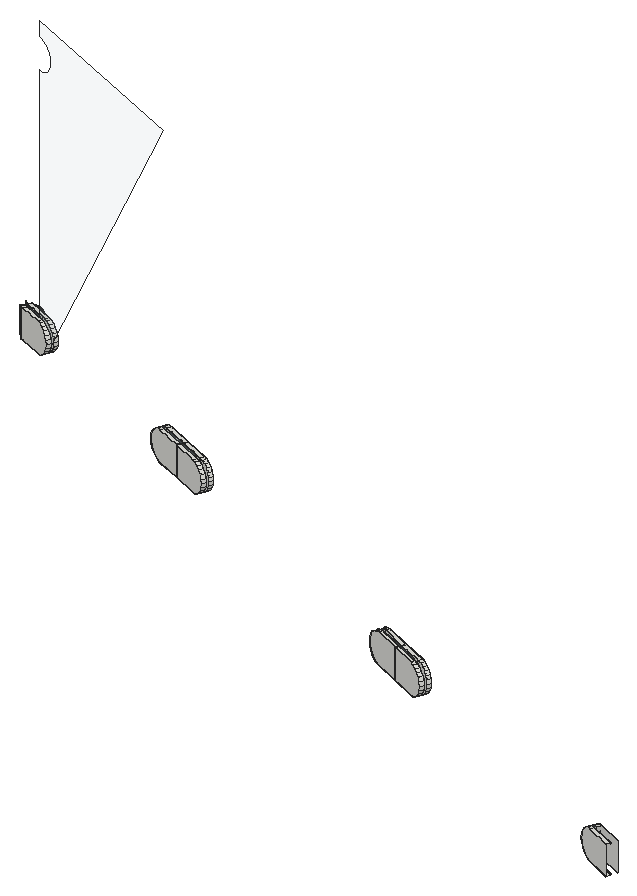
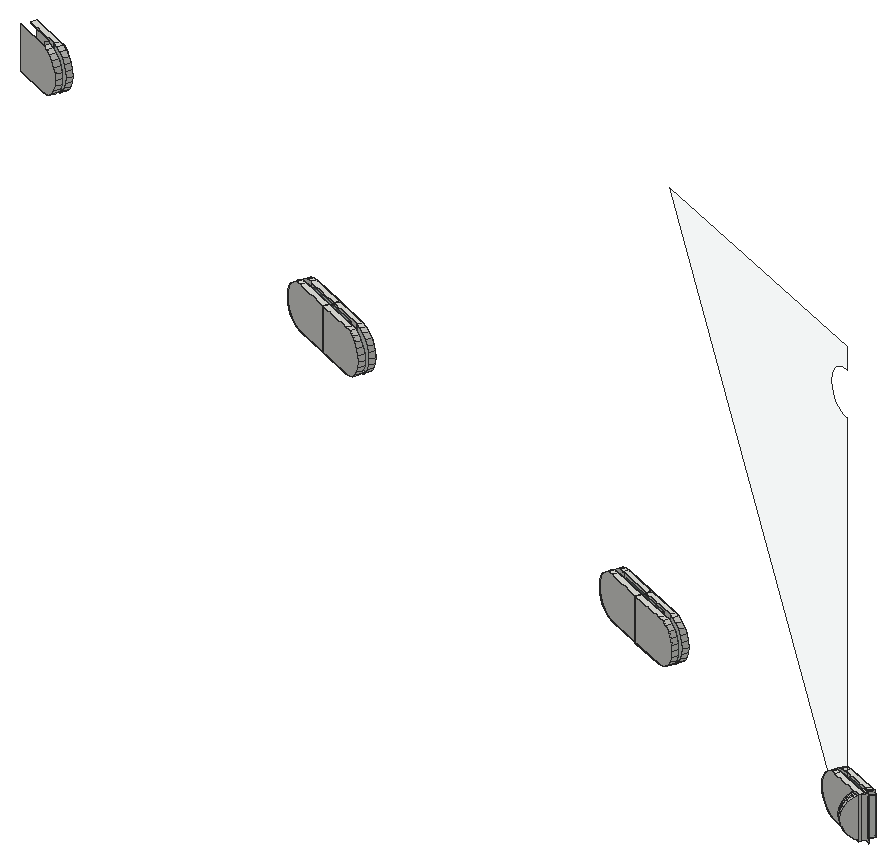
# SketchUp Ruby script. Lengths in inches.
U = 1.inch
M = Sketchup.active_model
def pt(a) = Geom::Point3d.new(a.map { |v| v * U })
def face(e, loops, mat)
  f = e.add_face(loops[0].map { |a| pt(a) })
  loops[1..].each { |l| e.add_face(l.map { |a| pt(a) }).erase! }
  f.material = f.back_material = mat if mat
  f
end
# faces: each face lists its corners as indices into pts; further lists are holes
def faces(e, pts, list, mat = nil) = list.each { |f| face(e, (f[0].is_a?(Array) ? f : [f]).map { |l| l.map { |i| pts[i] } }, mat) }
# xy, xz, yz: faces in a plane at the given z, y or x. An outline is a flat list of corners, or four numbers for a rectangle; further outlines are holes
def ring(l) = l.size == 4 ? [[l[0], l[1]], [l[2], l[1]], [l[2], l[3]], [l[0], l[3]]] : l.each_slice(2).to_a
def flat(e, list, mat, &to3) = list.each { |f| face(e, (f[0].is_a?(Array) ? f : [f]).map { |l| ring(l).map { |u, v| to3.(u, v) } }, mat) }
def xy(e, z, list, mat = nil) = flat(e, list, mat) { |x, y| [x, y, z] }
def xz(e, y, list, mat = nil) = flat(e, list, mat) { |x, z| [x, y, z] }
def yz(e, x, list, mat = nil) = flat(e, list, mat) { |y, z| [x, y, z] }
def lines(e, pts, list) = list.each { |a, b| e.add_line(pt(pts[a]), pt(pts[b])) }
# prism: a flat outline (further loops are holes) pulled along v
def prism(e, loops, v, mat = nil)
  f = face(e, loops, mat); d = Geom::Vector3d.new(v.map { |x| x * U })
  f.pushpull(f.normal.samedirection?(d) ? d.length : -d.length)
end
def box(e, o, s, mat = nil) = prism(e, [[o, [o[0] + s[0], o[1], o[2]], [o[0] + s[0], o[1] + s[1], o[2]], [o[0], o[1] + s[1], o[2]]]], [0, 0, s[2]], mat)
def at(x, y, z, deg = 0) = Geom::Transformation.translation(pt([x, y, z])) * Geom::Transformation.rotation(ORIGIN, Z_AXIS, deg.degrees)
def axes(o, x, y, z) = Geom::Transformation.new([*x, 0, *y, 0, *z, 0, *pt(o).to_a, 1])
def part(name) = M.definitions.add(name)
# library, detail: a bought-in or finely detailed component or shape, given as its bounding box
def library(name, o, s) = part(name).tap { |d| box(d.entities, o, s) }
def detail(e, o, s) = box(e.add_group.entities, o, s)
def put(e, d, t, mat = nil) = e.add_instance(d, t).tap { |i| i.material = mat if mat }
def group(e, t, mat = nil) = e.add_group.tap { |g| g.transformation = t; g.material = mat if mat }.entities
root = M.entities
M.materials.add("Glass_Safety_01").color = [204, 235, 244]
M.materials["Glass_Safety_01"].alpha = 0.1
xy(root,333,[[823.836,1099.203,822.031,1099.989,822.141,1100.242,823.946,1099.456],[802.031,1108.7,800.226,1109.486,800.336,1109.739,802.003,1109.013,802.141,1108.953],[802.22,1109.133,802.082,1109.193,800.415,1109.919,800.525,1110.172,802.33,1109.386],[800.226,1109.486,798.421,1110.272,798.531,1110.525,800.336,1109.739],[800.415,1109.919,798.61,1110.705,798.72,1110.958,800.525,1110.172],
  [777.687,1119.303,775.888,1120.086,775.994,1120.341,777.663,1119.614,777.797,1119.555],[777.876,1119.736,777.742,1119.794,776.071,1120.522,776.181,1120.775,777.986,1119.989],[775.888,1120.086,775.885,1120.087,775.882,1120.089,775.992,1120.341,775.994,1120.341],[775.882,1120.089,774.07,1120.841,774.176,1121.095,775.992,1120.341],[776.069,1120.523,774.251,1121.277,774.357,1121.532,776.175,1120.777],
  [760.716,1126.381,759.144,1127.034,759.32,1127.233,759.338,1127.252,760.627,1126.717,760.822,1126.636],[760.897,1126.818,760.702,1126.899,759.079,1127.572,759.184,1127.827,761.003,1127.072],[759.144,1127.034,758.951,1127.114,759.145,1127.332,759.265,1127.282,759.32,1127.233],[758.951,1127.114,758.898,1127.136,758.926,1127.204,759.068,1127.364,759.145,1127.332],[758.926,1127.204,759.003,1127.39,759.068,1127.364],
  [759.32,1127.233,759.265,1127.282,759.338,1127.252],[759.338,1127.252,759.265,1127.282,759.173,1127.364,759.195,1127.388,759.342,1127.257],[759.265,1127.282,759.145,1127.332,759.173,1127.364]])
xy(root,333.078,[[801.78,1109.11,800.336,1109.739,800.415,1109.919,801.859,1109.291],[800.336,1109.739,798.892,1110.368,798.971,1110.548,800.415,1109.919],[777.436,1119.713,775.994,1120.341,776.032,1120.432,776.071,1120.522,777.515,1119.893],[775.992,1120.341,774.539,1120.944,774.615,1121.126,776.069,1120.523,776.032,1120.432],[775.992,1120.341,776.032,1120.432,775.994,1120.341],
  [760.458,1126.787,759.068,1127.364,759.115,1127.416,759.041,1127.481,759.079,1127.572,760.533,1126.969],[758.875,1127.146,758.728,1127.277,758.968,1127.547,759.041,1127.481,759.003,1127.39,759.068,1127.364],[759.068,1127.364,759.003,1127.39,759.041,1127.481,759.115,1127.416]],"Glass_Safety_01")
xy(root,335.047,[[801.78,1109.11,801.859,1109.291,800.415,1109.919,800.336,1109.739],[800.336,1109.739,800.415,1109.919,798.971,1110.548,798.892,1110.368],[777.436,1119.713,777.515,1119.893,776.071,1120.522,776.032,1120.432,775.994,1120.341],[775.992,1120.341,776.032,1120.432,776.069,1120.523,774.615,1121.126,774.539,1120.944],[775.992,1120.341,775.994,1120.341,776.032,1120.432],
  [760.458,1126.787,760.533,1126.969,759.079,1127.572,759.041,1127.481,759.115,1127.416,759.068,1127.364],[758.875,1127.146,759.068,1127.364,759.003,1127.39,759.041,1127.481,758.968,1127.547,758.728,1127.277],[759.068,1127.364,759.115,1127.416,759.041,1127.481,759.003,1127.39]],"Glass_Safety_01")
xy(root,335.125,[[823.836,1099.203,823.946,1099.456,822.141,1100.242,822.031,1099.989],[802.031,1108.7,802.141,1108.953,802.003,1109.013,800.336,1109.739,800.226,1109.486],[802.22,1109.133,802.33,1109.386,800.525,1110.172,800.415,1109.919,802.082,1109.193],[800.226,1109.486,800.336,1109.739,798.531,1110.525,798.421,1110.272],[800.415,1109.919,800.525,1110.172,798.72,1110.958,798.61,1110.705],
  [777.687,1119.303,777.797,1119.555,777.663,1119.614,775.994,1120.341,775.888,1120.086],[777.876,1119.736,777.986,1119.989,776.181,1120.775,776.071,1120.522,777.742,1119.794],[775.888,1120.086,775.994,1120.341,775.992,1120.341,775.882,1120.089,775.885,1120.087],[775.882,1120.089,775.992,1120.341,774.176,1121.095,774.07,1120.841],[776.069,1120.523,776.175,1120.777,774.357,1121.532,774.251,1121.277],
  [760.716,1126.381,760.822,1126.636,760.627,1126.717,759.338,1127.252,759.32,1127.233,759.144,1127.034],[760.897,1126.818,761.003,1127.072,759.184,1127.827,759.079,1127.572,760.702,1126.899],[759.144,1127.034,759.32,1127.233,759.265,1127.282,759.145,1127.332,758.951,1127.114],[758.951,1127.114,759.145,1127.332,759.068,1127.364,758.926,1127.204,758.898,1127.136],[758.926,1127.204,759.068,1127.364,759.003,1127.39],
  [759.32,1127.233,759.338,1127.252,759.265,1127.282],[759.338,1127.252,759.342,1127.257,759.195,1127.388,759.173,1127.364,759.265,1127.282],[759.265,1127.282,759.173,1127.364,759.145,1127.332]])
xz(root,1120.341,[[775.992,333,775.994,333.078],[775.992,333.078,775.994,335.047],[775.992,333.078,775.994,335.125],[775.992,335.047,775.994,335.125]])
p = [[823.836,1099.203,335.125],[822.031,1099.989,335.125],[821.779,1100.099,335.089],[821.544,1100.202,334.983],[821.342,1100.29,334.814],[821.1875,1100.357,334.594],
  [821.09,1100.399,334.338],[821.057,1100.414,334.0625],[821.09,1100.399,333.787],[821.1875,1100.357,333.531],[821.342,1100.29,333.311],[821.544,1100.202,333.142],
  [821.779,1100.099,333.036],[822.031,1099.989,333],[823.836,1099.203,333],[823.946,1099.456,333],[822.141,1100.242,333],[822.141,1100.242,335.125],
  [823.946,1099.456,335.125],[823.946,1099.456,335.047],[822.502,1100.085,335.047],[822.502,1100.085,333.078],[823.946,1099.456,333.078],[822.33,1100.675,335.125],
  [824.135,1099.889,335.125],[824.135,1099.889,333],[822.33,1100.675,333],[822.078,1100.785,333.036],[821.843,1100.887,333.142],[821.641,1100.975,333.311],
  [821.486,1101.043,333.531],[821.389,1101.085,333.787],[821.355,1101.1,334.0625],[821.389,1101.085,334.338],[821.486,1101.043,334.594],[821.641,1100.975,334.814],
  [821.843,1100.887,334.983],[822.078,1100.785,335.089],[821.889,1100.352,333.036],[821.654,1100.454,333.142],[821.889,1100.352,335.089],[821.654,1100.454,334.983],
  [821.452,1100.542,334.814],[821.297,1100.61,334.594],[821.2,1100.652,334.338],[821.167,1100.667,334.0625],[821.2,1100.652,333.787],[821.297,1100.61,333.531],
  [821.452,1100.542,333.311],[822.22,1100.423,335.125],[822.22,1100.423,333],[821.968,1100.532,333.036],[821.733,1100.635,333.142],[821.531,1100.723,333.311],
  [821.376,1100.79,333.531],[821.279,1100.833,333.787],[821.245,1100.847,334.0625],[821.279,1100.833,334.338],[821.376,1100.79,334.594],[821.531,1100.723,334.814],
  [821.733,1100.635,334.983],[821.968,1100.532,335.089],[802.031,1108.7,335.125],[800.226,1109.486,335.125],[800.226,1109.486,333],[802.031,1108.7,333],
  [802.283,1108.59,333.036],[802.518,1108.488,333.142],[802.72,1108.4,333.311],[802.875,1108.333,333.531],[802.972,1108.29,333.787],[803.006,1108.276,334.0625],
  [802.972,1108.29,334.338],[802.875,1108.333,334.594],[802.72,1108.4,334.814],[802.518,1108.488,334.983],[802.283,1108.59,335.089],[802.141,1108.953,333],
  [802.003,1109.013,333],[802.003,1109.013,335.125],[802.141,1108.953,335.125],[802.393,1108.843,335.089],[802.628,1108.741,334.983],[802.83,1108.653,334.814],
  [802.985,1108.585,334.594],[803.082,1108.543,334.338],[803.116,1108.528,334.0625],[803.082,1108.543,333.787],[802.985,1108.585,333.531],[802.83,1108.653,333.311],
  [802.628,1108.741,333.142],[802.393,1108.843,333.036],[802.22,1109.133,335.125],[802.082,1109.193,335.125],[802.082,1109.193,333],[802.22,1109.133,333],
  [802.472,1109.023,333.036],[802.707,1108.921,333.142],[802.909,1108.833,333.311],[803.064,1108.766,333.531],[803.161,1108.723,333.787],[803.194,1108.709,334.0625],
  [803.161,1108.723,334.338],[803.064,1108.766,334.594],[802.909,1108.833,334.814],[802.707,1108.921,334.983],[802.472,1109.023,335.089],[802.582,1109.276,333.036],
  [802.817,1109.174,333.142],[800.336,1109.739,335.125],[800.336,1109.739,333],[800.336,1109.739,333.078],[801.78,1109.11,333.078],[801.78,1109.11,335.047],
  [800.336,1109.739,335.047],[800.525,1110.172,335.125],[802.33,1109.386,335.125],[802.582,1109.276,335.089],[802.817,1109.174,334.983],[803.019,1109.086,334.814],
  [803.174,1109.018,334.594],[803.271,1108.976,334.338],[803.304,1108.962,334.0625],[803.271,1108.976,333.787],[803.174,1109.018,333.531],[803.019,1109.086,333.311],
  [802.33,1109.386,333],[800.525,1110.172,333],[800.415,1109.919,333],[800.415,1109.919,335.125],[800.415,1109.919,335.047],[801.859,1109.291,335.047],
  [801.859,1109.291,333.078],[800.415,1109.919,333.078],[798.421,1110.272,335.125],[798.169,1110.382,335.089],[797.934,1110.484,334.983],[797.732,1110.572,334.814],
  [797.577,1110.64,334.594],[797.48,1110.682,334.338],[797.447,1110.697,334.0625],[797.48,1110.682,333.787],[797.577,1110.64,333.531],[797.732,1110.572,333.311],
  [797.934,1110.484,333.142],[798.169,1110.382,333.036],[798.421,1110.272,333],[798.531,1110.525,333],[798.531,1110.525,335.125],[798.892,1110.368,335.047],
  [798.892,1110.368,333.078],[798.61,1110.705,335.125],[798.61,1110.705,333],[798.971,1110.548,333.078],[798.971,1110.548,335.047],[798.72,1110.958,335.125],
  [798.72,1110.958,333],[798.468,1111.068,333.036],[798.233,1111.17,333.142],[798.031,1111.258,333.311],[797.876,1111.326,333.531],[797.779,1111.368,333.787],
  [797.746,1111.382,334.0625],[797.779,1111.368,334.338],[797.876,1111.326,334.594],[798.031,1111.258,334.814],[798.233,1111.17,334.983],[798.468,1111.068,335.089],
  [798.279,1110.635,333.036],[798.044,1110.737,333.142],[798.279,1110.635,335.089],[798.044,1110.737,334.983],[797.842,1110.825,334.814],[797.6875,1110.892,334.594],
  [797.59,1110.935,334.338],[797.557,1110.949,334.0625],[797.59,1110.935,333.787],[797.6875,1110.892,333.531],[797.842,1110.825,333.311],[798.358,1110.815,333.036],
  [798.123,1110.918,333.142],[797.921,1111.005,333.311],[797.766,1111.073,333.531],[797.669,1111.115,333.787],[797.636,1111.13,334.0625],[797.669,1111.115,334.338],
  [797.766,1111.073,334.594],[797.921,1111.005,334.814],[798.123,1110.918,334.983],[798.358,1110.815,335.089],[777.687,1119.303,335.125],[775.888,1120.086,335.125],
  [775.888,1120.086,333],[777.687,1119.303,333],[777.939,1119.193,333.036],[778.174,1119.09,333.142],[778.376,1119.003,333.311],[778.531,1118.935,333.531],
  [778.628,1118.893,333.787],[778.662,1118.878,334.0625],[778.628,1118.893,334.338],[778.531,1118.935,334.594],[778.376,1119.003,334.814],[778.174,1119.09,334.983],
  [777.939,1119.193,335.089],[777.797,1119.555,333],[777.663,1119.614,333],[777.663,1119.614,335.125],[777.797,1119.555,335.125],[778.049,1119.446,335.089],
  [778.284,1119.343,334.983],[778.486,1119.255,334.814],[778.641,1119.188,334.594],[778.738,1119.145,334.338],[778.772,1119.131,334.0625],[778.738,1119.145,333.787],
  [778.641,1119.188,333.531],[778.486,1119.255,333.311],[778.284,1119.343,333.142],[778.049,1119.446,333.036],[777.876,1119.736,335.125],[777.742,1119.794,335.125],
  [777.742,1119.794,333],[777.876,1119.736,333],[778.128,1119.626,333.036],[778.363,1119.524,333.142],[778.565,1119.436,333.311],[778.72,1119.368,333.531],
  [778.817,1119.326,333.787],[778.85,1119.311,334.0625],[778.817,1119.326,334.338],[778.72,1119.368,334.594],[778.565,1119.436,334.814],[778.363,1119.524,334.983],
  [778.128,1119.626,335.089],[778.238,1119.879,333.036],[778.473,1119.776,333.142],[775.994,1120.341,335.125],[775.994,1120.341,333],[775.994,1120.341,333.078],
  [777.436,1119.713,333.078],[777.436,1119.713,335.047],[775.994,1120.341,335.047],[776.181,1120.775,335.125],[777.986,1119.989,335.125],[778.238,1119.879,335.089],
  [778.473,1119.776,334.983],[778.675,1119.688,334.814],[778.83,1119.621,334.594],[778.927,1119.579,334.338],[778.96,1119.564,334.0625],[778.927,1119.579,333.787],
  [778.83,1119.621,333.531],[778.675,1119.688,333.311],[777.986,1119.989,333],[776.181,1120.775,333],[776.071,1120.522,333],[776.071,1120.522,335.125],
  [776.071,1120.522,335.047],[777.515,1119.893,335.047],[777.515,1119.893,333.078],[776.071,1120.522,333.078],[775.885,1120.087,335.125],[775.882,1120.089,335.125],
  [774.07,1120.841,335.125],[773.816,1120.946,335.089],[773.579,1121.044,334.983],[773.376,1121.129,334.814],[773.22,1121.193,334.594],[773.122,1121.234,334.338],
  [773.088,1121.248,334.0625],[773.122,1121.234,333.787],[773.22,1121.193,333.531],[773.376,1121.129,333.311],[773.579,1121.044,333.142],[773.816,1120.946,333.036],
  [774.07,1120.841,333],[775.882,1120.089,333],[775.885,1120.087,333],[775.992,1120.341,333.078],[775.992,1120.341,333],[775.992,1120.341,335.125],
  [775.992,1120.341,335.047],[774.176,1121.095,333],[774.176,1121.095,335.125],[774.539,1120.944,335.047],[774.539,1120.944,333.078],[776.069,1120.523,335.125],
  [774.251,1121.277,335.125],[774.251,1121.277,333],[776.069,1120.523,333],[776.069,1120.523,333.078],[774.615,1121.126,333.078],[774.615,1121.126,335.047],
  [776.069,1120.523,335.047],[776.175,1120.777,333],[776.175,1120.777,335.125],[774.357,1121.532,335.125],[774.357,1121.532,333],[774.103,1121.637,333.036],
  [773.866,1121.735,333.142],[773.662,1121.82,333.311],[773.506,1121.884,333.531],[773.408,1121.925,333.787],[773.375,1121.939,334.0625],[773.408,1121.925,334.338],
  [773.506,1121.884,334.594],[773.662,1121.82,334.814],[773.866,1121.735,334.983],[774.103,1121.637,335.089],[773.922,1121.201,333.036],[773.685,1121.299,333.142],
  [773.922,1121.201,335.089],[773.685,1121.299,334.983],[773.481,1121.383,334.814],[773.325,1121.448,334.594],[773.227,1121.489,334.338],[773.194,1121.503,334.0625],
  [773.227,1121.489,333.787],[773.325,1121.448,333.531],[773.481,1121.383,333.311],[773.997,1121.382,333.036],[773.76,1121.481,333.142],[773.557,1121.565,333.311],
  [773.401,1121.63,333.531],[773.303,1121.67,333.787],[773.269,1121.684,334.0625],[773.303,1121.67,334.338],[773.401,1121.63,334.594],[773.557,1121.565,334.814],
  [773.76,1121.481,334.983],[773.997,1121.382,335.089],[758.951,1127.114,335.125],[758.898,1127.136,335.125],[758.898,1127.136,333],[758.951,1127.114,333],
  [759.144,1127.034,333],[760.716,1126.381,333],[760.97,1126.276,333.036],[761.207,1126.178,333.142],[761.41,1126.093,333.311],[761.566,1126.029,333.531],
  [761.664,1125.988,333.787],[761.698,1125.974,334.0625],[761.664,1125.988,334.338],[761.566,1126.029,334.594],[761.41,1126.093,334.814],[761.207,1126.178,334.983],
  [760.97,1126.276,335.089],[760.716,1126.381,335.125],[759.144,1127.034,335.125],[761.773,1126.241,333.809],[761.433,1126.383,333.242],[761.3125,1126.432,333.142],
  [761.076,1126.531,333.036],[760.822,1126.636,333],[760.627,1126.717,333],[760.627,1126.717,335.125],[760.822,1126.636,335.125],[761.076,1126.531,335.089],
  [761.3125,1126.432,334.983],[761.516,1126.348,334.814],[761.672,1126.283,334.594],[761.77,1126.243,334.338],[761.803,1126.229,334.0625],[760.897,1126.818,335.125],
  [760.702,1126.899,335.125],[760.702,1126.899,333],[760.897,1126.818,333],[761.151,1126.712,333.036],[761.388,1126.614,333.142],[761.591,1126.53,333.311],
  [761.747,1126.465,333.531],[761.845,1126.424,333.787],[761.879,1126.41,334.0625],[761.845,1126.424,334.338],[761.747,1126.465,334.594],[761.591,1126.53,334.814],
  [761.388,1126.614,334.983],[761.151,1126.712,335.089],[761.257,1126.967,333.036],[761.494,1126.869,333.142],[759.338,1127.252,335.125],[759.338,1127.252,333],
  [759.265,1127.282,333],[759.145,1127.332,333],[759.068,1127.364,333],[759.003,1127.39,333],[759.003,1127.39,333.078],[759.068,1127.364,333.078],
  [760.458,1126.787,333.078],[760.458,1126.787,335.047],[759.068,1127.364,335.047],[759.003,1127.39,335.047],[759.003,1127.39,335.125],[759.068,1127.364,335.125],
  [759.145,1127.332,335.125],[759.265,1127.282,335.125],[759.184,1127.827,335.125],[761.003,1127.072,335.125],[761.257,1126.967,335.089],[761.494,1126.869,334.983],
  [761.697,1126.784,334.814],[761.853,1126.72,334.594],[761.951,1126.679,334.338],[761.984,1126.665,334.0625],[761.951,1126.679,333.787],[761.853,1126.72,333.531],
  [761.697,1126.784,333.311],[761.003,1127.072,333],[759.184,1127.827,333],[759.079,1127.572,333],[759.079,1127.572,335.125],[759.079,1127.572,335.047],
  [760.533,1126.969,335.047],[760.533,1126.969,333.078],[759.079,1127.572,333.078],[758.926,1127.204,333],[758.926,1127.204,335.125],[759.115,1127.416,333],
  [759.115,1127.416,333.078],[759.115,1127.416,335.047],[759.115,1127.416,335.125],[759.173,1127.364,335.125],[759.32,1127.233,335.125],[759.32,1127.233,333],
  [759.173,1127.364,333],[759.342,1127.257,335.125],[759.525,1127.463,335.089],[759.696,1127.654,334.983],[759.842,1127.819,334.814],[759.954,1127.945,334.594],
  [760.025,1128.024,334.338],[760.049,1128.051,334.0625],[760.025,1128.024,333.787],[759.954,1127.945,333.531],[759.842,1127.819,333.311],[759.696,1127.654,333.142],
  [759.525,1127.463,333.036],[759.342,1127.257,333],[759.378,1127.594,333.036],[759.195,1127.388,333],[758.989,1127.571,333],[759.172,1127.777,333.036],
  [759.319,1127.646,333.036],[759.136,1127.44,333],[758.968,1127.547,333.078],[758.968,1127.547,333],[758.762,1127.73,333],[758.762,1127.73,335.125],
  [758.968,1127.547,335.125],[758.968,1127.547,335.047],[758.989,1127.571,335.125],[759.172,1127.777,335.089],[759.343,1127.968,334.983],[759.489,1128.133,334.814],
  [759.602,1128.259,334.594],[759.672,1128.338,334.338],[759.696,1128.365,334.0625],[759.672,1128.338,333.787],[759.602,1128.259,333.531],[759.489,1128.133,333.311],
  [759.343,1127.968,333.142],[759.549,1127.785,333.142],[759.49,1127.837,333.142],[822.581,1100.265,335.047],[822.581,1100.265,333.078],[776.032,1120.432,335.047],
  [776.032,1120.432,333.078],[761.516,1126.348,333.311],[758.728,1127.277,333.078],[758.728,1127.277,335.047],[758.875,1127.146,335.047],[758.875,1127.146,333.078],
  [759.041,1127.481,335.047],[759.041,1127.481,333.078],[759.695,1127.949,333.311],[759.636,1128.002,333.311],[761.77,1126.243,333.787],[761.672,1126.283,333.531],
  [759.807,1128.076,333.531],[759.749,1128.128,333.531],[759.878,1128.155,333.787],[759.819,1128.207,333.787],[760.627,1126.717,351.283],[774.176,1121.095,354.511],
  [760.627,1126.717,354.511],[760.627,1126.717,353.409],[760.822,1126.636,353.409],[761.076,1126.531,353.373],[761.3125,1126.432,353.267],[761.516,1126.348,353.098],
  [761.672,1126.283,352.877],[761.77,1126.243,352.621],[761.803,1126.229,352.346],[761.77,1126.243,352.071],[761.672,1126.283,351.814],[761.516,1126.348,351.594],
  [761.3125,1126.432,351.425],[761.076,1126.531,351.319],[760.822,1126.636,351.283],[759.902,1128.182,334.0625],[759.843,1128.234,334.0625],[759.878,1128.155,334.338],
  [759.819,1128.207,334.338],[759.807,1128.076,334.594],[759.749,1128.128,334.594],[759.695,1127.949,334.814],[759.636,1128.002,334.814],[759.549,1127.785,334.983],
  [759.49,1127.837,334.983],[759.378,1127.594,335.089],[759.319,1127.646,335.089],[759.195,1127.388,335.125]]
faces(root,p,[[0,1,2,3,4,5,6,7,8,9,10,11,12,13,14],[15,16,17,18,19,20,21,22],[23,24,25,26,27,28,29,30,31,32,33,34,35,36,37],[38,16,13,12],[39,38,12,11],[50,51,27,26],[51,52,28,27],[62,63,64,65,66,67,68,69,70,71,72,73,74,75,76],
  [77,78,79,80,81,82,83,84,85,86,87,88,89,90,91],[91,90,67,66],[77,91,66,65],[92,93,94,95,96,97,98,99,100,101,102,103,104,105,106],[97,96,107,108],[109,79,78,110,111,112,113,114],[115,116,117,118,119,120,121,122,123,124,125,108,107,126,127],[96,95,126,107],
  [128,94,93,129,130,131,132,133],[63,134,135,136,137,138,139,140,141,142,143,144,145,146,64],[111,110,64,63,109,114],[110,147,148,109,114,149,150,111],[129,151,152,128,133,153,154,130],[128,133,130,129,115,127],[155,115,127,156,157,158,159,160,161,162,163,164,165,166,167],[168,147,146,145],
  [169,168,145,144],[152,179,157,156],[179,180,158,157],[190,191,192,193,194,195,196,197,198,199,200,201,202,203,204],[205,206,207,208,209,210,211,212,213,214,215,216,217,218,219],[219,218,195,194],[205,219,194,193],[220,221,222,223,224,225,226,227,228,229,230,231,232,233,234],
  [225,224,235,236],[237,207,206,238,239,240,241,242],[243,244,245,246,247,248,249,250,251,252,253,236,235,254,255],[224,223,254,235],[256,222,221,257,258,259,260,261],[191,262,263,264,265,266,267,268,269,270,271,272,273,274,275,276,277,278,192],[278,192,191,262,263,277],[279,280,277,263,281,282],
  [238,239,242,237,191,192],[280,283,284,281,282,285,286,279],[287,288,289,290,291,292,293,294],[291,290,295,296,287,294],[256,261,258,257,243,255],[297,296,295,298,299,300,301,302,303,304,305,306,307,308,309],[310,283,276,275],[311,310,275,274],
  [289,321,299,298],[321,322,300,299],[332,333,334,335,336,337,338,339,340,341,342,343,344,345,346,347,348,349,350],[354,353,339,338],[355,354,338,337],[365,366,367,368,369,370,371,372,373,374,375,376,377,378,379],[370,369,380,381],[382,357,356,383,384,385,386,387,388,389,390,391,392,393,394,395,396,397],
  [398,399,400,401,402,403,404,405,406,407,408,381,380,409,410],[369,368,409,380],[411,367,366,412,413,414,415,416],[388,387,417,334,333,418,394,393],[419,420,421,422,423,397,424,425,384,426],[383,425,424,382,427,428,429,430,431,432,433,434,435,436,437,438,439],[438,440,441,439],[442,443,444,445],
  [441,445,444,440],[446,447,448,449,450,451],[442,447,446,451,450,452,453,454,455,456,457,458,459,460,461,462,443],[437,463,440,438],[411,416,413,412,398,410],[443,462,464,444],[440,444,464,463],[48,39,11,10],
  [52,53,29,28],[90,89,68,67],[98,97,108,125],[178,169,144,143],[180,181,159,158],[218,217,196,195],[226,225,236,253],[285,282,279,286],
  [320,311,274,273],[322,323,301,300],[352,469,340,339,353],[371,370,381,408],[436,476,463,437],[462,461,477,464],[463,464,477,476],[351,478,479,469,352],
  [47,48,10,9],[53,54,30,29],[89,88,69,68],[99,98,125,124],[177,178,143,142],[181,182,160,159],[217,216,197,196],[227,226,253,252],
  [319,320,273,272],[323,324,302,301],[469,479,341,340],[372,371,408,407],[435,480,476,436],[476,477,481,480],[461,460,481,477],[46,47,9,8],
  [54,55,31,30],[88,87,70,69],[100,99,124,123],[176,177,142,141],[182,183,161,160],[216,215,198,197],[228,227,252,251],[318,319,272,271],
  [324,325,303,302],[479,478,342,341],[373,372,407,406],[434,482,480,435],[460,459,483,481],[480,481,483,482],[45,46,8,7],[55,56,32,31],
  [87,86,71,70],[101,100,123,122],[175,176,141,140],[183,184,162,161],[215,214,199,198],[229,228,251,250],[317,318,271,270],[325,326,304,303],
  [351,364,343,342,478],[374,373,406,405],[433,501,482,434],[459,458,502,483],[482,483,502,501],[44,45,7,6],[56,57,33,32],[86,85,72,71],
  [102,101,122,121],[174,175,140,139],[184,185,163,162],[214,213,200,199],[230,229,250,249],[316,317,270,269],[326,327,305,304],[364,363,344,343],
  [375,374,405,404],[432,503,501,433],[458,457,504,502],[501,502,504,503],[43,44,6,5],[57,58,34,33],[85,84,73,72],[103,102,121,120],
  [173,174,139,138],[185,186,164,163],[213,212,201,200],[231,230,249,248],[315,316,269,268],[327,328,306,305],[363,362,345,344],[376,375,404,403],
  [431,505,503,432],[457,456,506,504],[503,504,506,505],[42,43,5,4],[58,59,35,34],[84,83,74,73],[104,103,120,119],[172,173,138,137],
  [186,187,165,164],[212,211,202,201],[232,231,248,247],[314,315,268,267],[328,329,307,306],[362,361,346,345],[377,376,403,402],[430,507,505,431],
  [505,506,508,507],[456,455,508,506],[41,42,4,3],[59,60,36,35],[83,82,75,74],[105,104,119,118],[171,172,137,136],[187,188,166,165],
  [211,210,203,202],[233,232,247,246],[313,314,267,266],[329,330,308,307],[361,360,347,346],[378,377,402,401],[429,509,507,430],[455,454,510,508],
  [507,508,510,509],[40,41,3,2],[60,61,37,36],[82,81,76,75],[106,105,118,117],[170,171,136,135],[188,189,167,166],[210,209,204,203],
  [234,233,246,245],[312,313,266,265],[330,331,309,308],[360,359,348,347],[379,378,401,400],[428,511,509,429],[454,453,512,510],[509,510,512,511],
  [17,40,2,1],[61,49,23,37],[81,80,62,76],[92,106,117,116],[148,170,135,134],[189,151,155,167],[209,208,190,204],[220,234,245,244],
  [284,312,265,264],[331,288,297,309],[359,358,349,348],[365,379,400,399],[511,513,427,428],[452,513,511,512,453]])
faces(root,p,[[16,17,40,41,42,43,44,45,46,47,48,39,38],[49,50,51,52,53,54,55,56,57,58,59,60,61],[147,148,170,171,172,173,174,175,176,177,178,169,168],[151,152,179,180,181,182,183,184,185,186,187,188,189],[283,284,312,313,314,315,316,317,318,319,320,311,310],[288,289,321,322,323,324,325,326,327,328,329,330,331],[351,352,353,354,355,356,357,358,359,360,361,362,363,364],[21,20,465,466],
  [112,111,114,113],[132,131,113,112],[133,132,131,130],[111,150,149,114],[114,130,133,111],[153,133,130,154],[154,153,150,149],[242,241,240,239],
  [260,259,241,240],[261,260,259,258],[282,467,468,279],[468,467,242,239],[467,468,291,294],[261,468,467,258],[292,291,294,293],[292,286,285,293],
  [389,388,393,392,391,390],[415,414,391,390],[416,415,414,413],[470,471,472,473],[472,392,421,420,389,473],[446,470,471,451],[393,474,475,388],[475,474,421,420],
  [474,475,446,451],[416,475,474,413],[484,357,358,359,360,361,362,363,364,351,485,486,487,488,489,490,491,492,493,494,495,496,497,498,499,500]],"Glass_Safety_01")
lines(root,p,[[422,395],[386,419]])
